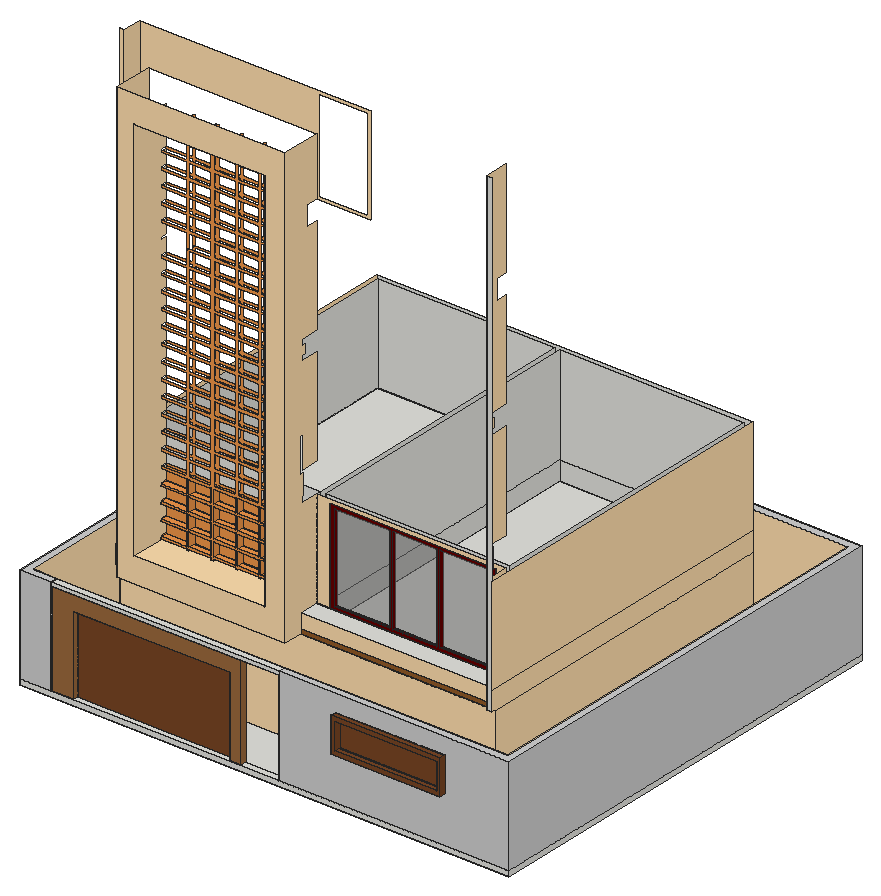
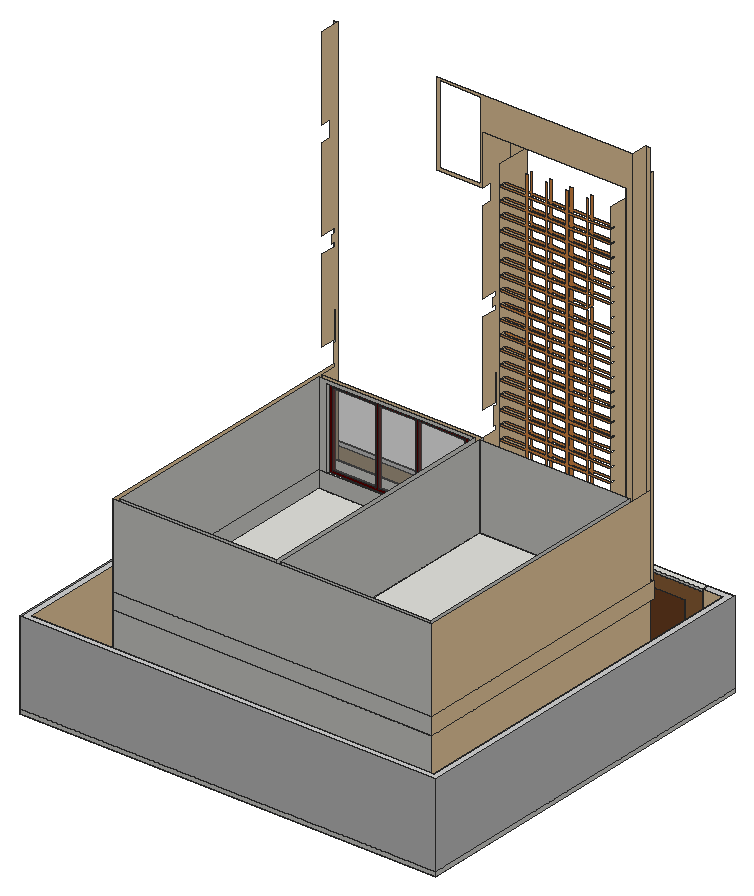
# SketchUp Ruby script. Lengths in inches.
U = 1.inch
M = Sketchup.active_model
def pt(a) = Geom::Point3d.new(a.map { |v| v * U })
def face(e, loops, mat)
  f = e.add_face(loops[0].map { |a| pt(a) })
  loops[1..].each { |l| e.add_face(l.map { |a| pt(a) }).erase! }
  f.material = f.back_material = mat if mat
  f
end
# faces: each face lists its corners as indices into pts; further lists are holes
def faces(e, pts, list, mat = nil) = list.each { |f| face(e, (f[0].is_a?(Array) ? f : [f]).map { |l| l.map { |i| pts[i] } }, mat) }
# xy, xz, yz: faces in a plane at the given z, y or x. An outline is a flat list of corners, or four numbers for a rectangle; further outlines are holes
def ring(l) = l.size == 4 ? [[l[0], l[1]], [l[2], l[1]], [l[2], l[3]], [l[0], l[3]]] : l.each_slice(2).to_a
def flat(e, list, mat, &to3) = list.each { |f| face(e, (f[0].is_a?(Array) ? f : [f]).map { |l| ring(l).map { |u, v| to3.(u, v) } }, mat) }
def xy(e, z, list, mat = nil) = flat(e, list, mat) { |x, y| [x, y, z] }
def xz(e, y, list, mat = nil) = flat(e, list, mat) { |x, z| [x, y, z] }
def yz(e, x, list, mat = nil) = flat(e, list, mat) { |y, z| [x, y, z] }
def lines(e, pts, list) = list.each { |a, b| e.add_line(pt(pts[a]), pt(pts[b])) }
# prism: a flat outline (further loops are holes) pulled along v
def prism(e, loops, v, mat = nil)
  f = face(e, loops, mat); d = Geom::Vector3d.new(v.map { |x| x * U })
  f.pushpull(f.normal.samedirection?(d) ? d.length : -d.length)
end
def box(e, o, s, mat = nil) = prism(e, [[o, [o[0] + s[0], o[1], o[2]], [o[0] + s[0], o[1] + s[1], o[2]], [o[0], o[1] + s[1], o[2]]]], [0, 0, s[2]], mat)
def at(x, y, z, deg = 0) = Geom::Transformation.translation(pt([x, y, z])) * Geom::Transformation.rotation(ORIGIN, Z_AXIS, deg.degrees)
def axes(o, x, y, z) = Geom::Transformation.new([*x, 0, *y, 0, *z, 0, *pt(o).to_a, 1])
def part(name) = M.definitions.add(name)
# library, detail: a bought-in or finely detailed component or shape, given as its bounding box
def library(name, o, s) = part(name).tap { |d| box(d.entities, o, s) }
def detail(e, o, s) = box(e.add_group.entities, o, s)
def put(e, d, t, mat = nil) = e.add_instance(d, t).tap { |i| i.material = mat if mat }
def group(e, t, mat = nil) = e.add_group.tap { |g| g.transformation = t; g.material = mat if mat }.entities
root = M.entities
M.materials.add("[0033_NavajoWhite]").color = [255, 222, 173]
M.materials.add("[Carrera Marble]1").color = [207, 207, 207]
M.materials.add("[Color A08]").color = [102, 0, 0]
M.materials.add("[Color M00]").color = [255, 255, 255]
M.materials.add("[Translucent Glass Gray]").color = [128, 128, 128]
M.materials["[Translucent Glass Gray]"].alpha = 0.5
M.materials.add("[Wood Floor Parquet]").color = [145, 89, 39]
M.materials.add("[Wood Floor]").color = [155, 105, 61]
M.materials.add("[Wood OSB]").color = [240, 151, 74]
M.materials.add("[Wood Veneer 01]").color = [120, 70, 37]
c1 = part("Group\#1")
xy(c1.entities,0,[[0,0,47.4375,3.5]],"[Color A08]")
xy(c1.entities,1.52,[[1.52,0,17.01,3.5],[17.01,0,18.02,3.5],[18.02,0,30.51,3.5],[30.51,0,31.52,3.5],[31.52,0,45.92,3.5]],"[Color A08]")
xy(c1.entities,45.92,[[1.52,0,17.01,3.5],[18.02,0,30.51,3.5],[31.52,0,45.92,3.5]],"[Color A08]")
xy(c1.entities,47.4375,[[0,0,47.4375,3.5]],"[Color A08]")
xz(c1.entities,0,[[[0,0,47.4375,47.4375],[1.52,1.52,1.52,45.92,17.01,45.92,17.01,1.52,18.02,1.52,18.02,45.92,30.51,45.92,30.51,1.52,31.52,1.52,31.52,45.92,45.92,45.92,45.92,1.52]]],"[Color A08]")
xz(c1.entities,3.5,[[[0,0,47.4375,47.4375],[1.52,1.52,45.92,1.52,45.92,45.92,31.52,45.92,31.52,1.52,30.51,1.52,30.51,45.92,18.02,45.92,18.02,1.52,17.01,1.52,17.01,45.92,1.52,45.92]]],"[Color A08]")
xz(c1.entities,3.5,[[1.52,1.52,17.01,45.92],[18.02,1.52,30.51,45.92],[31.52,1.52,45.92,45.92]],"[Translucent Glass Gray]")
yz(c1.entities,0,[[0,0,3.5,47.4375]],"[Color A08]")
yz(c1.entities,1.52,[[0,1.52,3.5,45.92]],"[Color A08]")
yz(c1.entities,17.01,[[0,1.52,3.5,45.92]],"[Color A08]")
yz(c1.entities,18.02,[[0,1.52,3.5,45.92]],"[Color A08]")
yz(c1.entities,30.51,[[0,1.52,3.5,45.92]],"[Color A08]")
yz(c1.entities,31.52,[[0,1.52,3.5,45.92]],"[Color A08]")
yz(c1.entities,45.92,[[0,1.52,3.5,45.92]],"[Color A08]")
yz(c1.entities,47.4375,[[0,0,3.5,47.4375]],"[Color A08]")
xy(root,0,[[0,7.125,600,547.125]])
xy(root,6,[[0,7.125,0,547.125,600,547.125,600,7.125,317.06,7.125,317.06,16.125,591,16.125,591,538.125,9,538.125,9,16.125,37.85,16.125,37.85,7.125],[37.85,7.125,64.78,8.875],[64.78,7.125,255.46,14.4375],[255.46,7.125,269.41,8.875],[269.41,7.125,317.06,16.125],
  [37.85,8.875,64.78,16.125],[255.46,8.875,269.41,16.125],[64.78,14.4375,68.8125,16.125],[68.8125,14.4375,74.0625,16.125],[74.0625,14.4375,255.46,16.125],
  [[9,16.125,591,538.125],[65.75,77,527.3125,471.125]],[[65.75,77,527.3125,471.125],[71.75,83,521.3125,465.125]],[71.75,83,521.3125,465.125]])
xy(root,62.92,[[386.9,0,520.95,7.125]],"[Wood Veneer 01]")
xy(root,67.53,[[391.52,0,516.33,7.125]],"[Wood Veneer 01]")
xy(root,100.6,[[391.52,0,516.33,7.125]],"[Wood Veneer 01]")
xy(root,102.44,[[64.78,14.4375,255.46,16.125]])
xy(root,102.44,[[64.78,8.875,255.46,14.4375]],"[Wood Floor]")
xy(root,105.21,[[386.9,0,520.95,7.125]],"[Wood Veneer 01]")
xy(root,120,[[71.75,83,521.3125,465.125]])
xy(root,122.125,[[37.85,7.125,269.41,8.875],[269.41,7.125,317.06,16.125],[37.85,8.875,269.41,16.125]])
xy(root,126,[[37.85,7.125,317.06,16.125],[[65.75,77,527.3125,471.125],[71.75,83,521.3125,83,521.3125,100.4375,289.0625,100.4375,289.0625,465.125,71.75,465.125,71.75,106.4375,289.0625,106.4375,289.0625,100.4375,71.75,100.4375],[295.0625,106.4375,521.3125,465.125]],[71.75,83,521.3125,100.4375],[71.75,106.4375,289.0625,465.125],[295.0625,106.4375,521.3125,465.125]])
xy(root,126,[[0,7.125,37.85,7.125,37.85,16.125,9,16.125,9,538.125,591,538.125,591,16.125,317.06,16.125,317.06,7.125,600,7.125,600,547.125,0,547.125]],"[Carrera Marble]1")
xy(root,127.5,[[82.77,51.6875,289.0625,71.3125]],"[Color M00]")
xy(root,127.5,[[65.75,71.3125,65.75,77,527.3125,77,527.3125,71.3125,521.3125,71.3125,521.3125,76.0625,289.0625,76.0625,289.0625,71.3125]],"[Wood Floor Parquet]")
xy(root,150,[[65.75,71.3125,71.75,77],[71.75,71.3125,82.77,83],[82.77,71.3125,263.87,83],[289.0625,76.0625,521.3125,100.4375],[71.75,83,82.77,100.4375],
  [82.77,83,263.87,100.4375],[263.87,83,289.0625,100.4375],[304.95,100.4375,509.02,106.4375],[71.75,106.4375,289.0625,465.125]])
xy(root,158.38,[[104.2,51.6875,263.87,51.6875,263.87,100.4375,226.62,100.4375,226.62,92.4375,224.24,92.4375,224.24,100.4375,198.13,100.4375,198.13,92.4375,195.99,92.4375,195.99,100.4375,169.17,100.4375,169.17,92.4375,165.875,92.4375,165.875,100.4375,139.19,100.4375,139.19,92.4375,136.74,92.4375,136.74,100.4375,104.2,100.4375]],"[0033_NavajoWhite]")
xy(root,158.38,[[136.74,92.4375,139.19,100.4375],[165.875,92.4375,169.17,100.4375],[195.99,92.4375,198.13,100.4375],[224.24,92.4375,226.62,100.4375]],"[Wood OSB]")
xy(root,159.59,[[104.2,92.4375,136.74,100.4375],[139.19,92.4375,165.875,100.4375],[169.17,92.4375,195.99,100.4375],[198.13,92.4375,224.24,100.4375],[226.62,92.4375,263.87,100.4375]],"[Wood OSB]")
xy(root,162.23,[[104.2,92.4375,136.74,100.4375],[139.19,92.4375,165.875,100.4375],[169.17,92.4375,195.99,100.4375],[198.13,92.4375,224.24,100.4375],[226.62,92.4375,263.87,100.4375]],"[Wood OSB]")
xy(root,178.9,[[104.2,92.4375,136.74,100.4375],[139.19,92.4375,165.875,100.4375],[169.17,92.4375,195.99,100.4375],[198.13,92.4375,224.24,100.4375],[226.62,92.4375,263.87,100.4375]],"[Wood OSB]")
xy(root,181.55,[[104.2,92.4375,136.74,100.4375],[139.19,92.4375,165.875,100.4375],[169.17,92.4375,195.99,100.4375],[198.13,92.4375,224.24,100.4375],[226.62,92.4375,263.87,100.4375]],"[Wood OSB]")
xy(root,198.22,[[104.2,92.4375,136.74,100.4375],[139.19,92.4375,165.875,100.4375],[169.17,92.4375,195.99,100.4375],[198.13,92.4375,224.24,100.4375],[226.62,92.4375,263.87,100.4375]],"[Wood OSB]")
xy(root,200.86,[[104.2,92.4375,136.74,100.4375],[139.19,92.4375,165.875,100.4375],[169.17,92.4375,195.99,100.4375],[198.13,92.4375,224.24,100.4375],[226.62,92.4375,263.87,100.4375]],"[Wood OSB]")
xy(root,217.53,[[104.2,92.4375,136.74,100.4375],[139.19,92.4375,165.875,100.4375],[169.17,92.4375,195.99,100.4375],[198.13,92.4375,224.24,100.4375],[226.62,92.4375,263.87,100.4375]],"[Wood OSB]")
xy(root,220.17,[[104.2,92.4375,136.74,100.4375],[139.19,92.4375,165.875,100.4375],[169.17,92.4375,195.99,100.4375],[198.13,92.4375,224.24,100.4375],[226.62,92.4375,263.87,100.4375]],"[Wood OSB]")
xz(root,0,[[[386.9,62.92,520.95,105.21],[391.52,67.53,516.33,100.6]]],"[Wood Veneer 01]")
xz(root,7.125,[[0,0,600,6],[37.85,122.125,317.06,126]])
xz(root,7.125,[[0,6,37.85,126],[[317.06,6,600,126],[386.9,62.92,520.95,105.21]]],"[Carrera Marble]1")
xz(root,7.125,[[[386.9,62.92,520.95,105.21],[391.52,67.53,516.33,100.6]],[391.52,67.53,516.33,100.6]],"[Wood Veneer 01]")
xz(root,8.875,[[37.85,6,64.78,6,64.78,102.44,255.46,102.44,255.46,6,269.41,6,269.41,122.125,37.85,122.125]],"[Wood Floor]")
xz(root,14.4375,[[64.78,6,255.46,102.44]],"[Wood Veneer 01]")
xz(root,16.125,[[37.85,122.125,317.06,126]])
xz(root,16.125,[[9,6,37.85,126],[317.06,6,591,126]],"[0033_NavajoWhite]")
xz(root,16.125,[[37.85,6,37.85,122.125,269.41,122.125,269.41,6,255.46,6,255.46,102.44,64.78,102.44,64.78,6]],"[Wood Floor]")
xz(root,16.125,[[64.78,6,255.46,102.44]],"[Wood Veneer 01]")
xz(root,51.6875,[[[82.77,127.5,289.0625,665.86],[104.2,158.38,263.87,633.42]]],"[0033_NavajoWhite]")
xz(root,71.3125,[[82.77,127.5,263.87,150],[521.3125,127.5,527.3125,714.125]])
xz(root,71.3125,[[65.75,127.5,82.77,150]],"[0033_NavajoWhite]")
xz(root,76.0625,[[289.0625,132.93,521.3125,150]],"[0033_NavajoWhite]")
xz(root,76.0625,[[289.0625,127.5,521.3125,132.93]],"[Wood Floor Parquet]")
xz(root,77,[[65.75,6,527.3125,126],[65.75,150,71.75,714.125]],"[0033_NavajoWhite]")
xz(root,77,[[65.75,126,527.3125,127.5]],"[Wood Floor Parquet]")
xz(root,83,[[71.75,6,521.3125,120],[71.75,120,521.3125,126]])
xz(root,92.4375,[[[136.74,158.38,139.19,158.38,139.19,159.59,165.875,159.59,165.875,158.38,169.17,158.38,169.17,159.59,195.99,159.59,195.99,158.38,198.13,158.38,198.13,159.59,224.24,159.59,224.24,158.38,226.62,158.38,226.62,159.59,263.87,159.59,263.87,162.23,226.62,162.23,226.62,178.9,263.87,178.9,263.87,181.55,226.62,181.55,226.62,198.22,263.87,198.22,263.87,200.86,226.62,200.86,226.62,217.53,263.87,217.53,263.87,220.17,226.62,220.17,226.62,236.84,263.87,236.84,263.87,239.48,226.62,239.48,226.62,256.15,263.87,256.15,263.87,258.8,226.62,258.8,226.62,275.47,263.87,275.47,263.87,278.11,226.62,278.11,226.62,294.78,263.87,294.78,263.87,297.42,226.62,297.42,226.62,314.09,263.87,314.09,263.87,316.73,226.62,316.73,226.62,333.4,263.87,333.4,263.87,336.05,226.62,336.05,226.62,352.72,263.87,352.72,263.87,355.36,226.62,355.36,226.62,372.03,263.87,372.03,263.87,374.67,226.62,374.67,226.62,391.34,263.87,391.34,263.87,393.98,226.62,393.98,226.62,410.65,263.87,410.65,263.87,413.3,226.62,413.3,226.62,429.97,263.87,429.97,263.87,432.61,226.62,432.61,226.62,449.28,263.87,449.28,263.87,451.92,226.62,451.92,226.62,468.59,263.87,468.59,263.87,471.23,226.62,471.23,226.62,487.9,263.87,487.9,263.87,490.55,226.62,490.55,226.62,507.22,263.87,507.22,263.87,509.86,226.62,509.86,226.62,526.53,263.87,526.53,263.87,529.17,226.62,529.17,226.62,545.84,263.87,545.84,263.87,548.48,226.62,548.48,226.62,565.15,263.87,565.15,263.87,567.8,226.62,567.8,226.62,584.47,263.87,584.47,263.87,587.11,226.62,587.11,226.62,603.78,263.87,603.78,263.87,606.42,226.62,606.42,226.62,633.42,224.24,633.42,224.24,606.42,198.13,606.42,198.13,633.42,195.99,633.42,195.99,606.42,169.17,606.42,169.17,633.42,165.875,633.42,165.875,606.42,139.19,606.42,139.19,633.42,136.74,633.42,136.74,606.42,104.2,606.42,104.2,603.78,136.74,603.78,136.74,587.11,104.2,587.11,104.2,584.47,136.74,584.47,136.74,567.8,104.2,567.8,104.2,565.15,136.74,565.15,136.74,548.48,104.2,548.48,104.2,545.84,136.74,545.84,136.74,529.17,104.2,529.17,104.2,526.53,136.74,526.53,136.74,509.86,104.2,509.86,104.2,507.22,136.74,507.22,136.74,490.55,139.19,490.55,139.19,507.22,165.875,507.22,165.875,490.55,139.19,490.55,139.19,487.9,165.875,487.9,165.875,471.23,139.19,471.23,139.19,487.9,136.74,487.9,136.74,471.23,104.2,471.23,104.2,468.59,136.74,468.59,136.74,451.92,104.2,451.92,104.2,449.28,136.74,449.28,136.74,432.61,104.2,432.61,104.2,429.97,136.74,429.97,136.74,413.3,104.2,413.3,104.2,410.65,136.74,410.65,136.74,393.98,104.2,393.98,104.2,391.34,136.74,391.34,136.74,374.67,104.2,374.67,104.2,372.03,136.74,372.03,136.74,355.36,104.2,355.36,104.2,352.72,136.74,352.72,136.74,336.05,104.2,336.05,104.2,333.4,136.74,333.4,136.74,316.73,104.2,316.73,104.2,314.09,136.74,314.09,136.74,297.42,104.2,297.42,104.2,294.78,136.74,294.78,136.74,278.11,104.2,278.11,104.2,275.47,136.74,275.47,136.74,258.8,104.2,258.8,104.2,256.15,136.74,256.15,136.74,239.48,104.2,239.48,104.2,236.84,136.74,236.84,136.74,220.17,104.2,220.17,104.2,217.53,136.74,217.53,136.74,200.86,104.2,200.86,104.2,198.22,136.74,198.22,136.74,181.55,104.2,181.55,104.2,178.9,136.74,178.9,136.74,162.23,104.2,162.23,104.2,159.59,136.74,159.59],[169.17,162.23,195.99,178.9],[169.17,490.55,195.99,507.22],[169.17,432.61,195.99,449.28],[169.17,258.8,195.99,275.47],[169.17,200.86,195.99,217.53],[169.17,278.11,195.99,294.78],[169.17,297.42,195.99,314.09],[169.17,316.73,195.99,333.4],[169.17,336.05,195.99,352.72],[169.17,355.36,195.99,372.03],[169.17,374.67,195.99,391.34],[169.17,393.98,195.99,410.65],[169.17,413.3,195.99,429.97],[169.17,451.92,195.99,468.59],[169.17,471.23,195.99,487.9],[169.17,509.86,195.99,526.53],[169.17,529.17,195.99,545.84],[169.17,548.48,195.99,565.15],[169.17,239.48,195.99,256.15],[169.17,181.55,195.99,198.22],[169.17,220.17,195.99,236.84],[169.17,567.8,195.99,584.47],[169.17,587.11,195.99,603.78],[139.19,162.23,165.875,178.9],[139.19,587.11,165.875,603.78],[139.19,548.48,165.875,565.15],[139.19,567.8,165.875,584.47],[139.19,509.86,165.875,526.53],[139.19,451.92,165.875,468.59],[139.19,393.98,165.875,410.65],[139.19,374.67,165.875,391.34],[139.19,355.36,165.875,372.03],[139.19,336.05,165.875,352.72],[139.19,297.42,165.875,314.09],[139.19,316.73,165.875,333.4],[139.19,200.86,165.875,217.53],[139.19,278.11,165.875,294.78],[139.19,258.8,165.875,275.47],[139.19,432.61,165.875,449.28],[139.19,413.3,165.875,429.97],[139.19,529.17,165.875,545.84],[139.19,181.55,165.875,198.22],[139.19,239.48,165.875,256.15],[139.19,220.17,165.875,236.84],[198.13,451.92,224.24,468.59],[198.13,162.23,224.24,178.9],[198.13,548.48,224.24,565.15],[198.13,509.86,224.24,526.53],[198.13,490.55,224.24,507.22],[198.13,471.23,224.24,487.9],[198.13,432.61,224.24,449.28],[198.13,393.98,224.24,410.65],[198.13,374.67,224.24,391.34],[198.13,355.36,224.24,372.03],[198.13,316.73,224.24,333.4],[198.13,297.42,224.24,314.09],[198.13,220.17,224.24,236.84],[198.13,258.8,224.24,275.47],[198.13,278.11,224.24,294.78],[198.13,336.05,224.24,352.72],[198.13,413.3,224.24,429.97],[198.13,529.17,224.24,545.84],[198.13,200.86,224.24,217.53],[198.13,181.55,224.24,198.22],[198.13,239.48,224.24,256.15],[198.13,587.11,224.24,603.78],[198.13,567.8,224.24,584.47]]],"[Wood OSB]")
xz(root,100.4375,[[104.2,101.65,263.87,104.3],[104.2,120.97,263.87,123.61],[[71.75,126,289.0625,150],[104.2,140.28,263.87,142.92]],[289.0625,126,521.3125,150],[104.2,140.28,263.87,142.92],
  [104.2,158.38,136.74,159.59],[139.19,158.38,165.875,159.59],[169.17,158.38,195.99,159.59],[198.13,158.38,224.24,159.59],[226.62,158.38,263.87,159.59]])
xz(root,100.4375,[[[71.75,150,82.77,150,82.77,665.86,289.0625,665.86,289.0625,594.125,355.82,594.125,355.82,714.125,71.75,714.125],[292.08,597.4375,351.27,711.0625]],[289.0625,150,304.95,150,304.95,265.4375,509.02,265.4375,509.02,150,521.3125,150,521.3125,270,289.0625,270]],"[0033_NavajoWhite]")
xz(root,100.4375,[[[136.74,158.38,136.74,159.59,104.2,159.59,104.2,162.23,136.74,162.23,136.74,178.9,104.2,178.9,104.2,181.55,136.74,181.55,136.74,198.22,104.2,198.22,104.2,200.86,136.74,200.86,136.74,217.53,104.2,217.53,104.2,220.17,136.74,220.17,136.74,236.84,104.2,236.84,104.2,239.48,136.74,239.48,136.74,256.15,104.2,256.15,104.2,258.8,136.74,258.8,136.74,275.47,104.2,275.47,104.2,278.11,136.74,278.11,136.74,294.78,104.2,294.78,104.2,297.42,136.74,297.42,136.74,314.09,104.2,314.09,104.2,316.73,136.74,316.73,136.74,333.4,104.2,333.4,104.2,336.05,136.74,336.05,136.74,352.72,104.2,352.72,104.2,355.36,136.74,355.36,136.74,372.03,104.2,372.03,104.2,374.67,136.74,374.67,136.74,391.34,104.2,391.34,104.2,393.98,136.74,393.98,136.74,410.65,104.2,410.65,104.2,413.3,136.74,413.3,136.74,429.97,104.2,429.97,104.2,432.61,136.74,432.61,136.74,449.28,104.2,449.28,104.2,451.92,136.74,451.92,136.74,468.59,104.2,468.59,104.2,471.23,136.74,471.23,136.74,487.9,139.19,487.9,139.19,471.23,165.875,471.23,165.875,487.9,139.19,487.9,139.19,490.55,165.875,490.55,165.875,507.22,139.19,507.22,139.19,490.55,136.74,490.55,136.74,507.22,104.2,507.22,104.2,509.86,136.74,509.86,136.74,526.53,104.2,526.53,104.2,529.17,136.74,529.17,136.74,545.84,104.2,545.84,104.2,548.48,136.74,548.48,136.74,565.15,104.2,565.15,104.2,567.8,136.74,567.8,136.74,584.47,104.2,584.47,104.2,587.11,136.74,587.11,136.74,603.78,104.2,603.78,104.2,606.42,136.74,606.42,136.74,633.42,139.19,633.42,139.19,606.42,165.875,606.42,165.875,633.42,169.17,633.42,169.17,606.42,195.99,606.42,195.99,633.42,198.13,633.42,198.13,606.42,224.24,606.42,224.24,633.42,226.62,633.42,226.62,606.42,263.87,606.42,263.87,603.78,226.62,603.78,226.62,587.11,263.87,587.11,263.87,584.47,226.62,584.47,226.62,567.8,263.87,567.8,263.87,565.15,226.62,565.15,226.62,548.48,263.87,548.48,263.87,545.84,226.62,545.84,226.62,529.17,263.87,529.17,263.87,526.53,226.62,526.53,226.62,509.86,263.87,509.86,263.87,507.22,226.62,507.22,226.62,490.55,263.87,490.55,263.87,487.9,226.62,487.9,226.62,471.23,263.87,471.23,263.87,468.59,226.62,468.59,226.62,451.92,263.87,451.92,263.87,449.28,226.62,449.28,226.62,432.61,263.87,432.61,263.87,429.97,226.62,429.97,226.62,413.3,263.87,413.3,263.87,410.65,226.62,410.65,226.62,393.98,263.87,393.98,263.87,391.34,226.62,391.34,226.62,374.67,263.87,374.67,263.87,372.03,226.62,372.03,226.62,355.36,263.87,355.36,263.87,352.72,226.62,352.72,226.62,336.05,263.87,336.05,263.87,333.4,226.62,333.4,226.62,316.73,263.87,316.73,263.87,314.09,226.62,314.09,226.62,297.42,263.87,297.42,263.87,294.78,226.62,294.78,226.62,278.11,263.87,278.11,263.87,275.47,226.62,275.47,226.62,258.8,263.87,258.8,263.87,256.15,226.62,256.15,226.62,239.48,263.87,239.48,263.87,236.84,226.62,236.84,226.62,220.17,263.87,220.17,263.87,217.53,226.62,217.53,226.62,200.86,263.87,200.86,263.87,198.22,226.62,198.22,226.62,181.55,263.87,181.55,263.87,178.9,226.62,178.9,226.62,162.23,263.87,162.23,263.87,159.59,226.62,159.59,226.62,158.38,224.24,158.38,224.24,159.59,198.13,159.59,198.13,158.38,195.99,158.38,195.99,159.59,169.17,159.59,169.17,158.38,165.875,158.38,165.875,159.59,139.19,159.59,139.19,158.38],[169.17,162.23,195.99,178.9],[169.17,490.55,195.99,507.22],[169.17,432.61,195.99,449.28],[169.17,258.8,195.99,275.47],[169.17,200.86,195.99,217.53],[169.17,278.11,195.99,294.78],[169.17,297.42,195.99,314.09],[169.17,316.73,195.99,333.4],[169.17,336.05,195.99,352.72],[169.17,355.36,195.99,372.03],[169.17,374.67,195.99,391.34],[169.17,393.98,195.99,410.65],[169.17,413.3,195.99,429.97],[169.17,451.92,195.99,468.59],[169.17,471.23,195.99,487.9],[169.17,509.86,195.99,526.53],[169.17,529.17,195.99,545.84],[169.17,548.48,195.99,565.15],[169.17,239.48,195.99,256.15],[169.17,181.55,195.99,198.22],[169.17,220.17,195.99,236.84],[169.17,567.8,195.99,584.47],[169.17,587.11,195.99,603.78],[139.19,162.23,165.875,178.9],[139.19,587.11,165.875,603.78],[139.19,548.48,165.875,565.15],[139.19,567.8,165.875,584.47],[139.19,509.86,165.875,526.53],[139.19,451.92,165.875,468.59],[139.19,393.98,165.875,410.65],[139.19,374.67,165.875,391.34],[139.19,355.36,165.875,372.03],[139.19,336.05,165.875,352.72],[139.19,297.42,165.875,314.09],[139.19,316.73,165.875,333.4],[139.19,200.86,165.875,217.53],[139.19,278.11,165.875,294.78],[139.19,258.8,165.875,275.47],[139.19,432.61,165.875,449.28],[139.19,413.3,165.875,429.97],[139.19,529.17,165.875,545.84],[139.19,181.55,165.875,198.22],[139.19,239.48,165.875,256.15],[139.19,220.17,165.875,236.84],[198.13,451.92,224.24,468.59],[198.13,162.23,224.24,178.9],[198.13,548.48,224.24,565.15],[198.13,509.86,224.24,526.53],[198.13,490.55,224.24,507.22],[198.13,471.23,224.24,487.9],[198.13,432.61,224.24,449.28],[198.13,393.98,224.24,410.65],[198.13,374.67,224.24,391.34],[198.13,355.36,224.24,372.03],[198.13,316.73,224.24,333.4],[198.13,297.42,224.24,314.09],[198.13,220.17,224.24,236.84],[198.13,258.8,224.24,275.47],[198.13,278.11,224.24,294.78],[198.13,336.05,224.24,352.72],[198.13,413.3,224.24,429.97],[198.13,529.17,224.24,545.84],[198.13,200.86,224.24,217.53],[198.13,181.55,224.24,198.22],[198.13,239.48,224.24,256.15],[198.13,587.11,224.24,603.78],[198.13,567.8,224.24,584.47]],[104.2,162.23,136.74,178.9],[139.19,162.23,165.875,178.9],[169.17,162.23,195.99,178.9],[198.13,162.23,224.24,178.9],
  [226.62,162.23,263.87,178.9],[104.2,181.55,136.74,198.22],[139.19,181.55,165.875,198.22],[169.17,181.55,195.99,198.22],[198.13,181.55,224.24,198.22],
  [226.62,181.55,263.87,198.22],[104.2,200.86,136.74,217.53],[139.19,200.86,165.875,217.53],[169.17,200.86,195.99,217.53],[198.13,200.86,224.24,217.53],
  [226.62,200.86,263.87,217.53],[104.2,220.17,136.74,236.84],[139.19,220.17,165.875,236.84],[169.17,220.17,195.99,236.84],[198.13,220.17,224.24,236.84],
  [226.62,220.17,263.87,236.84]],"[Wood OSB]")
xz(root,106.4375,[[71.75,126,289.0625,150],[295.0625,126,521.3125,150],[71.75,150,289.0625,270],[295.0625,150,295.0625,270,521.3125,270,521.3125,150,509.02,150,509.02,265.4375,304.95,265.4375,304.95,150]])
xz(root,465.125,[[71.75,6,521.3125,120],[71.75,120,97.53,126],[97.53,120,118.4,126],[71.75,126,97.53,150],[97.53,126,118.4,150],
  [118.4,126,289.0625,150],[295.0625,126,521.3125,150],[71.75,150,289.0625,270],[295.0625,150,521.3125,270]])
xz(root,471.125,[[65.75,6,527.3125,126],[65.75,126,527.3125,150],[65.75,150,527.3125,270]])
xz(root,538.125,[[9,6,591,126]],"[0033_NavajoWhite]")
xz(root,547.125,[[0,0,600,6]])
xz(root,547.125,[[0,6,600,126]],"[Carrera Marble]1")
yz(root,0,[[7.125,0,547.125,6]])
yz(root,0,[[7.125,6,547.125,126]],"[Carrera Marble]1")
yz(root,9,[[16.125,6,538.125,126]],"[0033_NavajoWhite]")
yz(root,37.85,[[7.125,6,8.875,122.125],[8.875,6,16.125,122.125],[7.125,122.125,16.125,126]])
yz(root,64.78,[[14.4375,6,16.125,102.44]])
yz(root,64.78,[[8.875,6,14.4375,102.44]],"[Wood Floor]")
yz(root,65.75,[[77,6,471.125,126],[77,126,77,127.5,71.3125,127.5,71.3125,150,471.125,150,471.125,126],[77,150,471.125,270]],"[0033_NavajoWhite]")
yz(root,71.75,[[83,6,465.125,120],[83,126,100.4375,150],[106.4375,126,465.125,150],[106.4375,150,465.125,270]])
yz(root,71.75,[[77,150,100.4375,714.125]],"[0033_NavajoWhite]")
yz(root,82.77,[[51.6875,127.5,51.6875,665.86,100.4375,665.86,100.4375,150,71.3125,150,71.3125,127.5]],"[0033_NavajoWhite]")
yz(root,104.2,[[51.6875,158.38,100.4375,158.38,100.4375,159.59,92.4375,159.59,92.4375,162.23,100.4375,162.23,100.4375,178.9,92.4375,178.9,92.4375,181.55,100.4375,181.55,100.4375,198.22,92.4375,198.22,92.4375,200.86,100.4375,200.86,100.4375,217.53,92.4375,217.53,92.4375,220.17,100.4375,220.17,100.4375,236.84,92.4375,236.84,92.4375,239.48,100.4375,239.48,100.4375,256.15,92.4375,256.15,92.4375,258.8,100.4375,258.8,100.4375,275.47,92.4375,275.47,92.4375,278.11,100.4375,278.11,100.4375,294.78,92.4375,294.78,92.4375,297.42,100.4375,297.42,100.4375,314.09,92.4375,314.09,92.4375,316.73,100.4375,316.73,100.4375,333.4,92.4375,333.4,92.4375,336.05,100.4375,336.05,100.4375,352.72,92.4375,352.72,92.4375,355.36,100.4375,355.36,100.4375,372.03,92.4375,372.03,92.4375,374.67,100.4375,374.67,100.4375,391.34,92.4375,391.34,92.4375,393.98,100.4375,393.98,100.4375,410.65,92.4375,410.65,92.4375,413.3,100.4375,413.3,100.4375,429.97,92.4375,429.97,92.4375,432.61,100.4375,432.61,100.4375,449.28,92.4375,449.28,92.4375,451.92,100.4375,451.92,100.4375,468.59,92.4375,468.59,92.4375,471.23,100.4375,471.23,100.4375,487.9,92.4375,487.9,92.4375,490.55,100.4375,490.55,100.4375,507.22,92.4375,507.22,92.4375,509.86,100.4375,509.86,100.4375,526.53,92.4375,526.53,92.4375,529.17,100.4375,529.17,100.4375,545.84,92.4375,545.84,92.4375,548.48,100.4375,548.48,100.4375,565.15,92.4375,565.15,92.4375,567.8,100.4375,567.8,100.4375,584.47,92.4375,584.47,92.4375,587.11,100.4375,587.11,100.4375,603.78,92.4375,603.78,92.4375,606.42,100.4375,606.42,100.4375,633.42,51.6875,633.42]],"[0033_NavajoWhite]")
yz(root,104.2,[[92.4375,159.59,100.4375,162.23],[92.4375,178.9,100.4375,181.55],[92.4375,198.22,100.4375,200.86],[92.4375,217.53,100.4375,220.17]],"[Wood OSB]")
yz(root,136.74,[[92.4375,158.38,100.4375,159.59],[92.4375,162.23,100.4375,178.9],[92.4375,181.55,100.4375,198.22],[92.4375,200.86,100.4375,217.53],[92.4375,220.17,100.4375,236.84]],"[Wood OSB]")
yz(root,139.19,[[92.4375,158.38,100.4375,159.59],[92.4375,162.23,100.4375,178.9],[92.4375,181.55,100.4375,198.22],[92.4375,200.86,100.4375,217.53],[92.4375,220.17,100.4375,236.84]],"[Wood OSB]")
yz(root,165.875,[[92.4375,158.38,100.4375,159.59],[92.4375,162.23,100.4375,178.9],[92.4375,181.55,100.4375,198.22],[92.4375,200.86,100.4375,217.53],[92.4375,220.17,100.4375,236.84]],"[Wood OSB]")
yz(root,169.17,[[92.4375,158.38,100.4375,159.59],[92.4375,162.23,100.4375,178.9],[92.4375,181.55,100.4375,198.22],[92.4375,200.86,100.4375,217.53],[92.4375,220.17,100.4375,236.84]],"[Wood OSB]")
yz(root,195.99,[[92.4375,158.38,100.4375,159.59],[92.4375,162.23,100.4375,178.9],[92.4375,181.55,100.4375,198.22],[92.4375,200.86,100.4375,217.53],[92.4375,220.17,100.4375,236.84]],"[Wood OSB]")
yz(root,198.13,[[92.4375,158.38,100.4375,159.59],[92.4375,162.23,100.4375,178.9],[92.4375,181.55,100.4375,198.22],[92.4375,200.86,100.4375,217.53],[92.4375,220.17,100.4375,236.84]],"[Wood OSB]")
yz(root,224.24,[[92.4375,158.38,100.4375,159.59],[92.4375,162.23,100.4375,178.9],[92.4375,181.55,100.4375,198.22],[92.4375,200.86,100.4375,217.53],[92.4375,220.17,100.4375,236.84]],"[Wood OSB]")
yz(root,226.62,[[92.4375,158.38,100.4375,159.59],[92.4375,162.23,100.4375,178.9],[92.4375,181.55,100.4375,198.22],[92.4375,200.86,100.4375,217.53],[92.4375,220.17,100.4375,236.84]],"[Wood OSB]")
yz(root,255.46,[[14.4375,6,16.125,102.44]])
yz(root,255.46,[[8.875,6,14.4375,102.44]],"[Wood Floor]")
yz(root,263.87,[[51.6875,158.38,51.6875,633.42,100.4375,633.42,100.4375,606.42,92.4375,606.42,92.4375,603.78,100.4375,603.78,100.4375,587.11,92.4375,587.11,92.4375,584.47,100.4375,584.47,100.4375,567.8,92.4375,567.8,92.4375,565.15,100.4375,565.15,100.4375,548.48,92.4375,548.48,92.4375,545.84,100.4375,545.84,100.4375,529.17,92.4375,529.17,92.4375,526.53,100.4375,526.53,100.4375,509.86,92.4375,509.86,92.4375,507.22,100.4375,507.22,100.4375,490.55,92.4375,490.55,92.4375,487.9,100.4375,487.9,100.4375,471.23,92.4375,471.23,92.4375,468.59,100.4375,468.59,100.4375,451.92,92.4375,451.92,92.4375,449.28,100.4375,449.28,100.4375,432.61,92.4375,432.61,92.4375,429.97,100.4375,429.97,100.4375,413.3,92.4375,413.3,92.4375,410.65,100.4375,410.65,100.4375,393.98,92.4375,393.98,92.4375,391.34,100.4375,391.34,100.4375,374.67,92.4375,374.67,92.4375,372.03,100.4375,372.03,100.4375,355.36,92.4375,355.36,92.4375,352.72,100.4375,352.72,100.4375,336.05,92.4375,336.05,92.4375,333.4,100.4375,333.4,100.4375,316.73,92.4375,316.73,92.4375,314.09,100.4375,314.09,100.4375,297.42,92.4375,297.42,92.4375,294.78,100.4375,294.78,100.4375,278.11,92.4375,278.11,92.4375,275.47,100.4375,275.47,100.4375,258.8,92.4375,258.8,92.4375,256.15,100.4375,256.15,100.4375,239.48,92.4375,239.48,92.4375,236.84,100.4375,236.84,100.4375,220.17,92.4375,220.17,92.4375,217.53,100.4375,217.53,100.4375,200.86,92.4375,200.86,92.4375,198.22,100.4375,198.22,100.4375,181.55,92.4375,181.55,92.4375,178.9,100.4375,178.9,100.4375,162.23,92.4375,162.23,92.4375,159.59,100.4375,159.59,100.4375,158.38]],"[0033_NavajoWhite]")
yz(root,263.87,[[92.4375,159.59,100.4375,162.23],[92.4375,178.9,100.4375,181.55],[92.4375,198.22,100.4375,200.86],[92.4375,217.53,100.4375,220.17]],"[Wood OSB]")
yz(root,269.41,[[8.875,6,16.125,122.125]],"[Wood Floor]")
yz(root,289.0625,[[100.4375,126,106.4375,150],[106.4375,126,465.125,150],[100.4375,150,106.4375,270],[106.4375,150,465.125,270]])
yz(root,289.0625,[[51.6875,127.5,76.0625,127.5,76.0625,150,100.4375,150,100.4375,270,77,270,77,277,79.6875,277,79.6875,302.125,74.75,302.125,74.75,344.375,78.69,344.375,78.69,306,100.4375,306,100.4375,426.125,77,426.125,77,432.1875,82.1875,432.1875,82.1875,443.4375,77,443.4375,77,450.125,100.4375,450.125,100.4375,570.125,85.8125,570.125,85.8125,594.125,100.4375,594.125,100.4375,665.86,51.6875,665.86]],"[0033_NavajoWhite]")
yz(root,295.0625,[[106.4375,126,465.125,150],[106.4375,150,465.125,270]])
yz(root,304.95,[[100.4375,150,106.4375,265.4375]])
yz(root,317.06,[[7.125,6,16.125,122.125]],"[Carrera Marble]1")
yz(root,386.9,[[0,62.92,7.125,105.21]],"[Wood Veneer 01]")
yz(root,391.52,[[0,67.53,7.125,100.6]],"[Wood Veneer 01]")
yz(root,509.02,[[100.4375,150,106.4375,265.4375]])
yz(root,516.33,[[0,67.53,7.125,100.6]],"[Wood Veneer 01]")
yz(root,520.95,[[0,62.92,7.125,105.21]],"[Wood Veneer 01]")
yz(root,521.3125,[[83,6,465.125,120],[83,126,100.4375,150],[106.4375,126,465.125,150],[106.4375,150,465.125,270]])
yz(root,521.3125,[[71.3125,127.5,71.3125,714.125,100.4375,714.125,100.4375,594.125,85.8125,594.125,85.8125,570.125,100.4375,570.125,100.4375,450.125,77,450.125,77,443.4375,82.1875,443.4375,82.1875,432.1875,77,432.1875,77,426.125,100.4375,426.125,100.4375,306,78.69,306,78.69,344.375,74.75,344.375,74.75,302.125,79.6875,302.125,79.6875,277,77,277,77,270,100.4375,270,100.4375,150,76.0625,150,76.0625,127.5]],"[0033_NavajoWhite]")
yz(root,527.3125,[[77,6,471.125,126],[77,126,471.125,126,471.125,150,71.3125,150,71.3125,127.5,77,127.5],[71.3125,150,471.125,270]],"[0033_NavajoWhite]")
yz(root,591,[[16.125,6,538.125,126]],"[0033_NavajoWhite]")
yz(root,600,[[7.125,0,547.125,6]])
yz(root,600,[[7.125,6,547.125,126]],"[Carrera Marble]1")
p = [[521.3125,465.125,120],[521.3125,465.125,126]]
lines(root,p,[[0,1]])
put(root,c1,axes([304.95,100.54,150],[4.30188,0,0],[0,0.97,0],[0,0,2.43351]))
